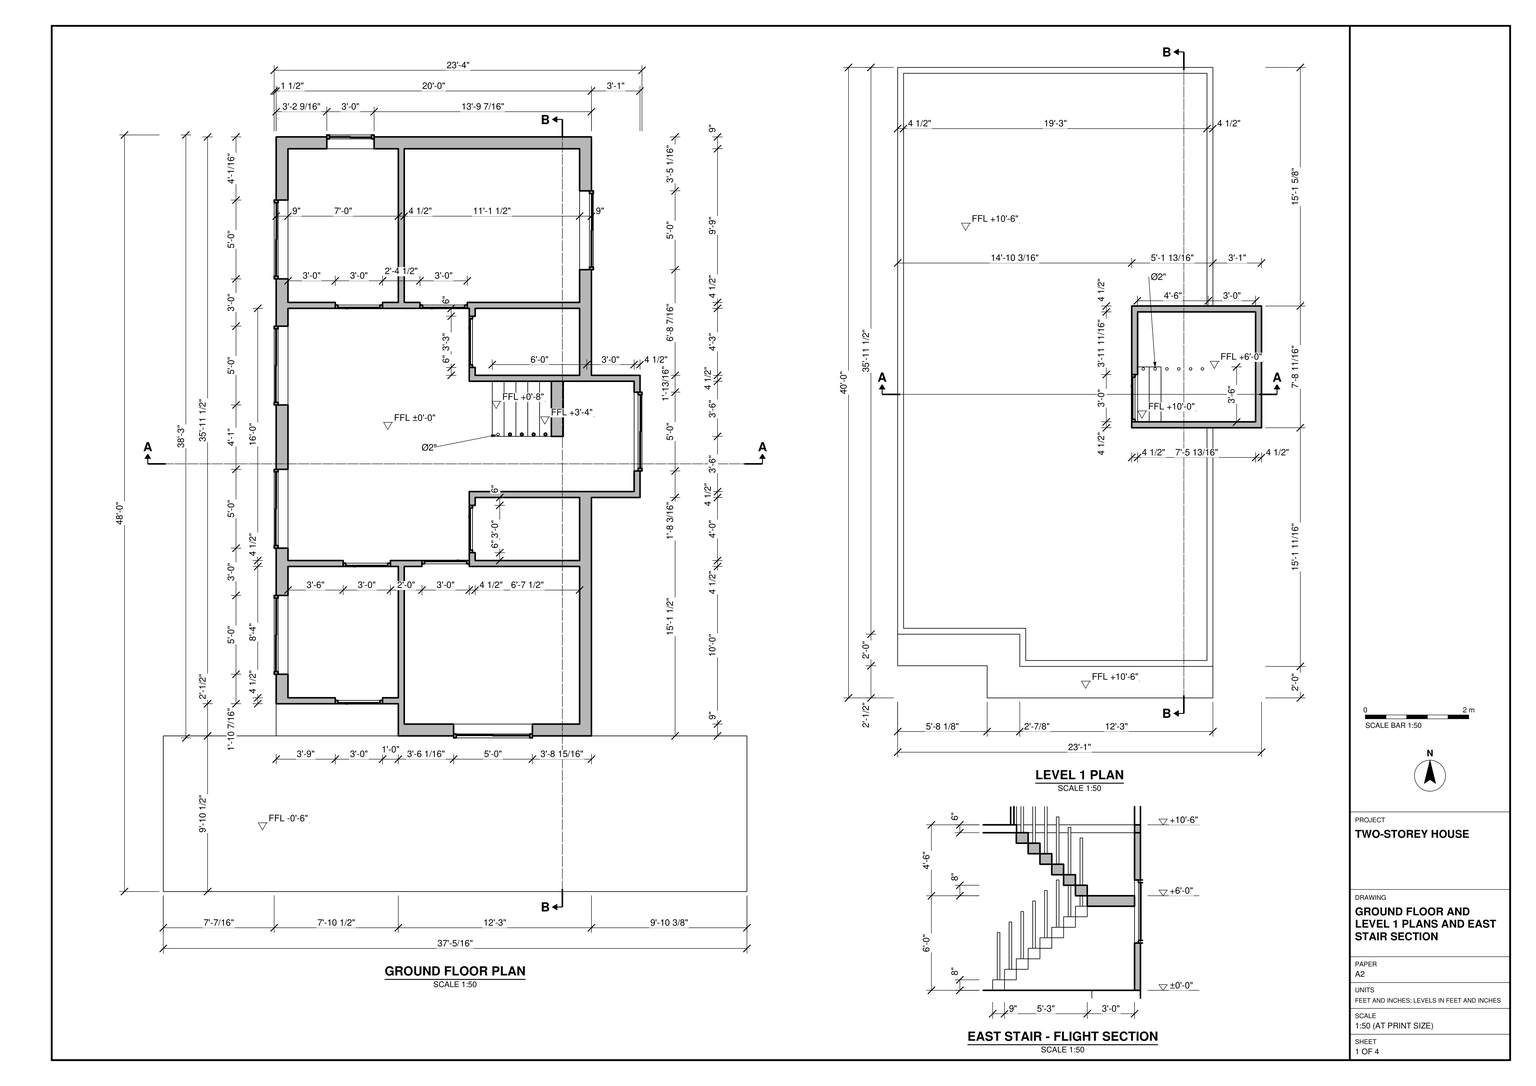
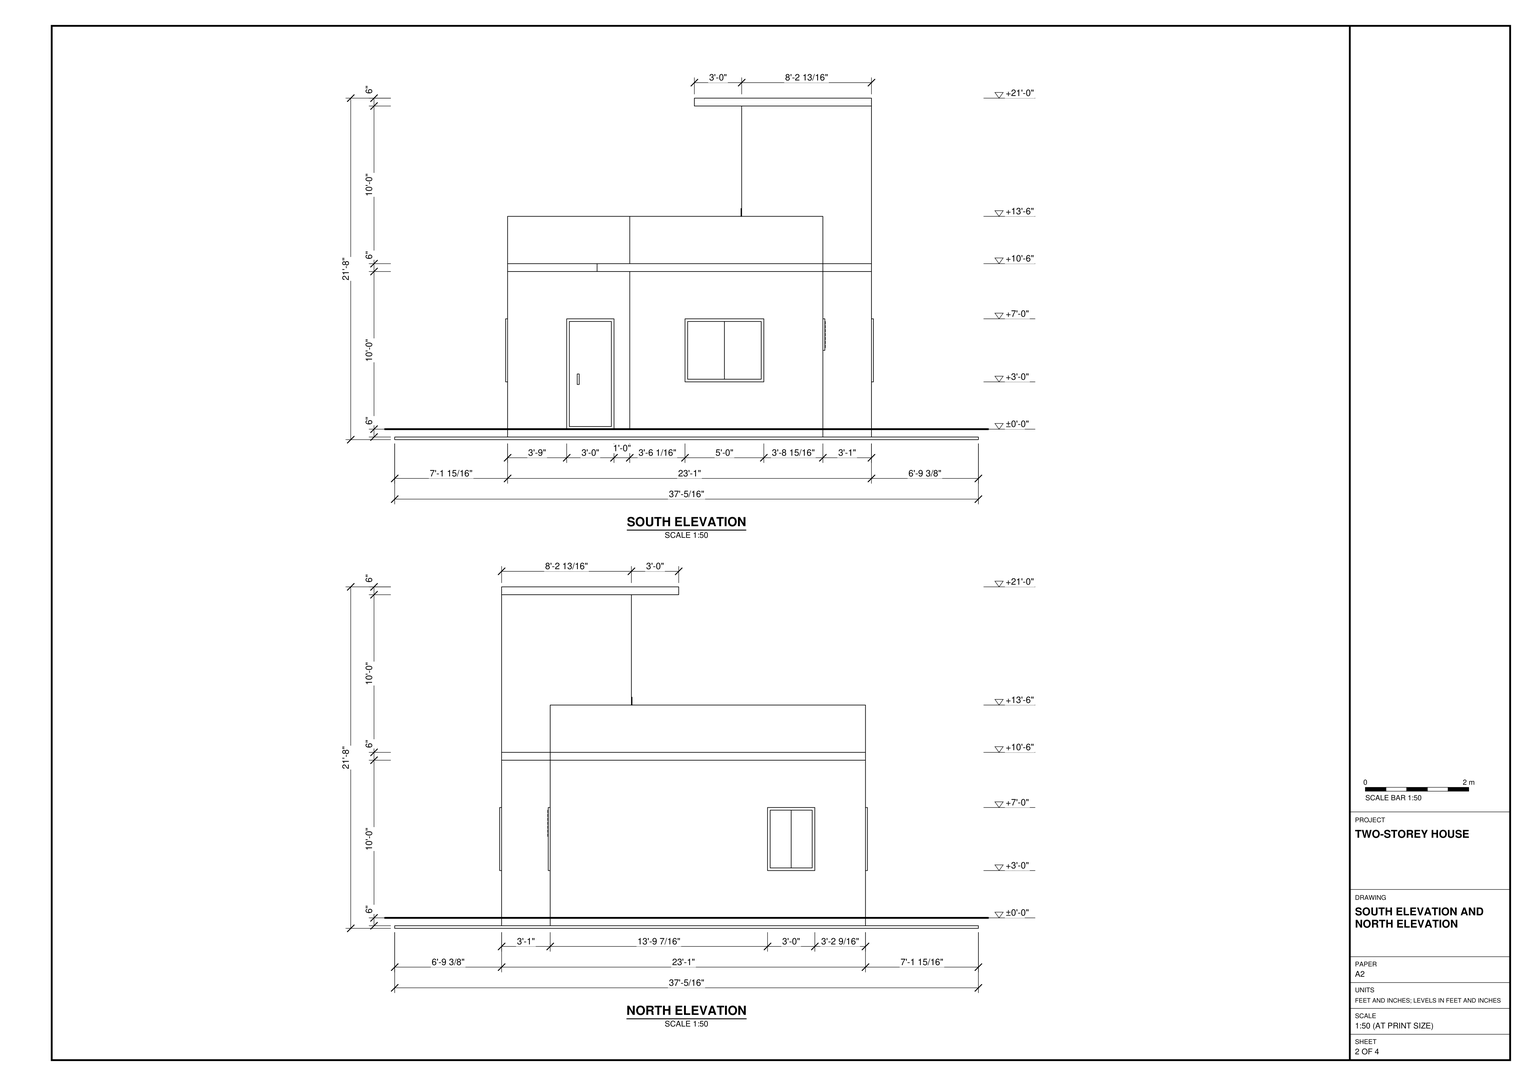
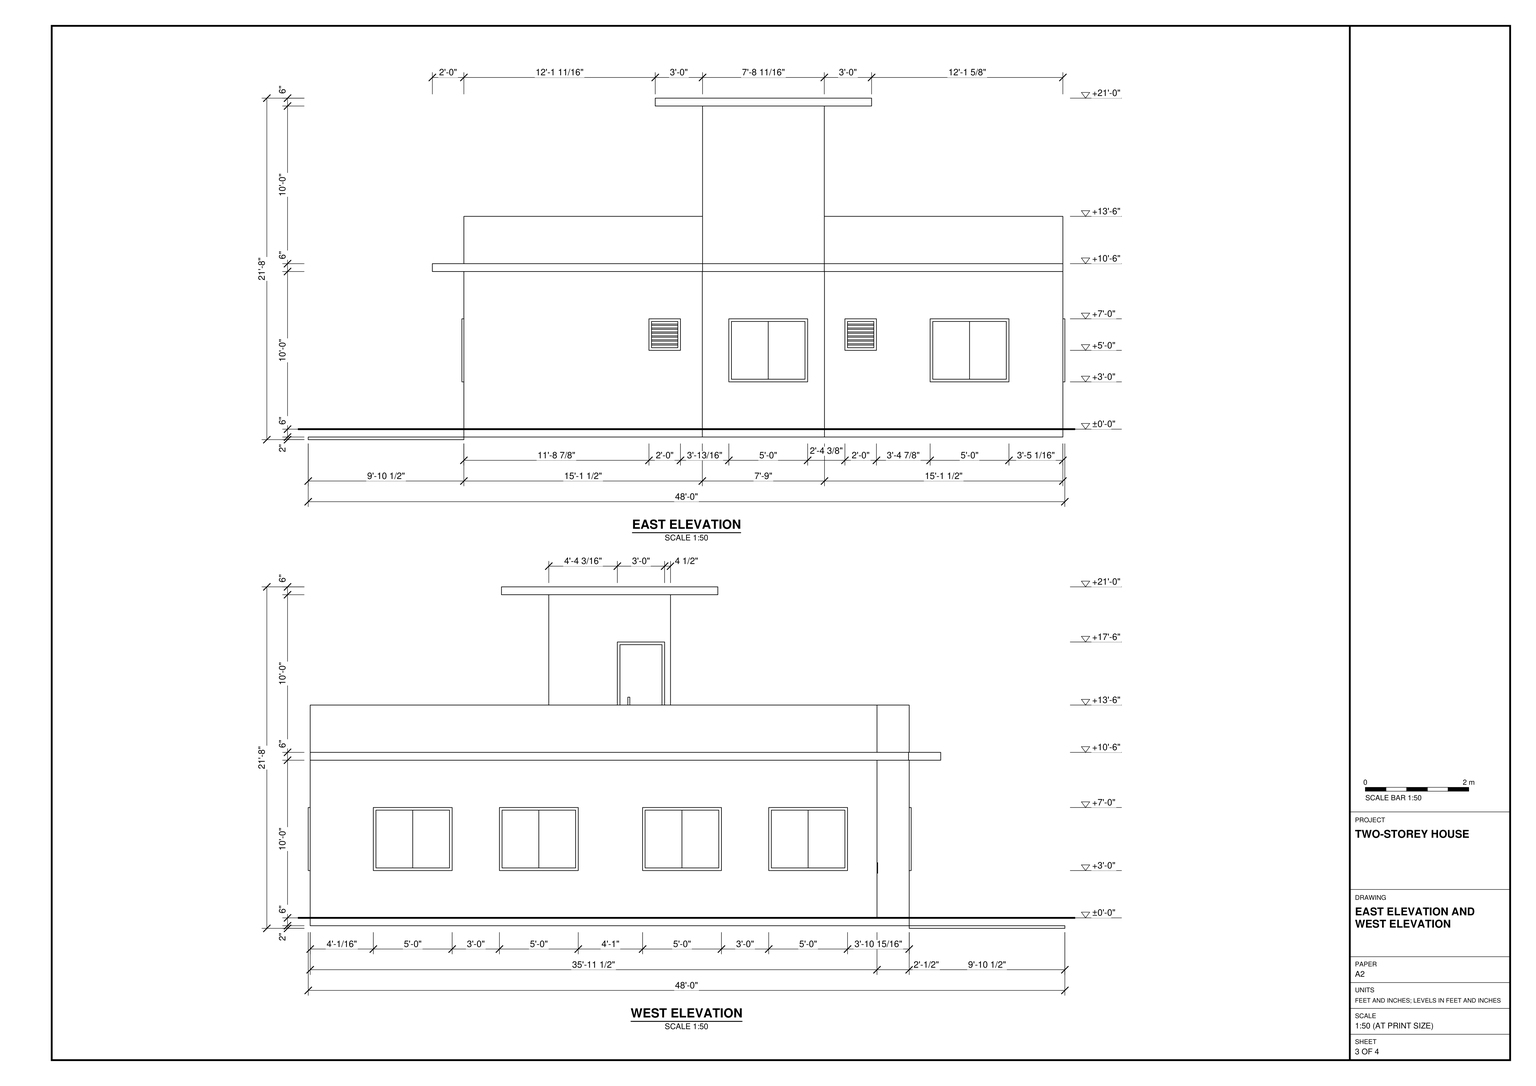
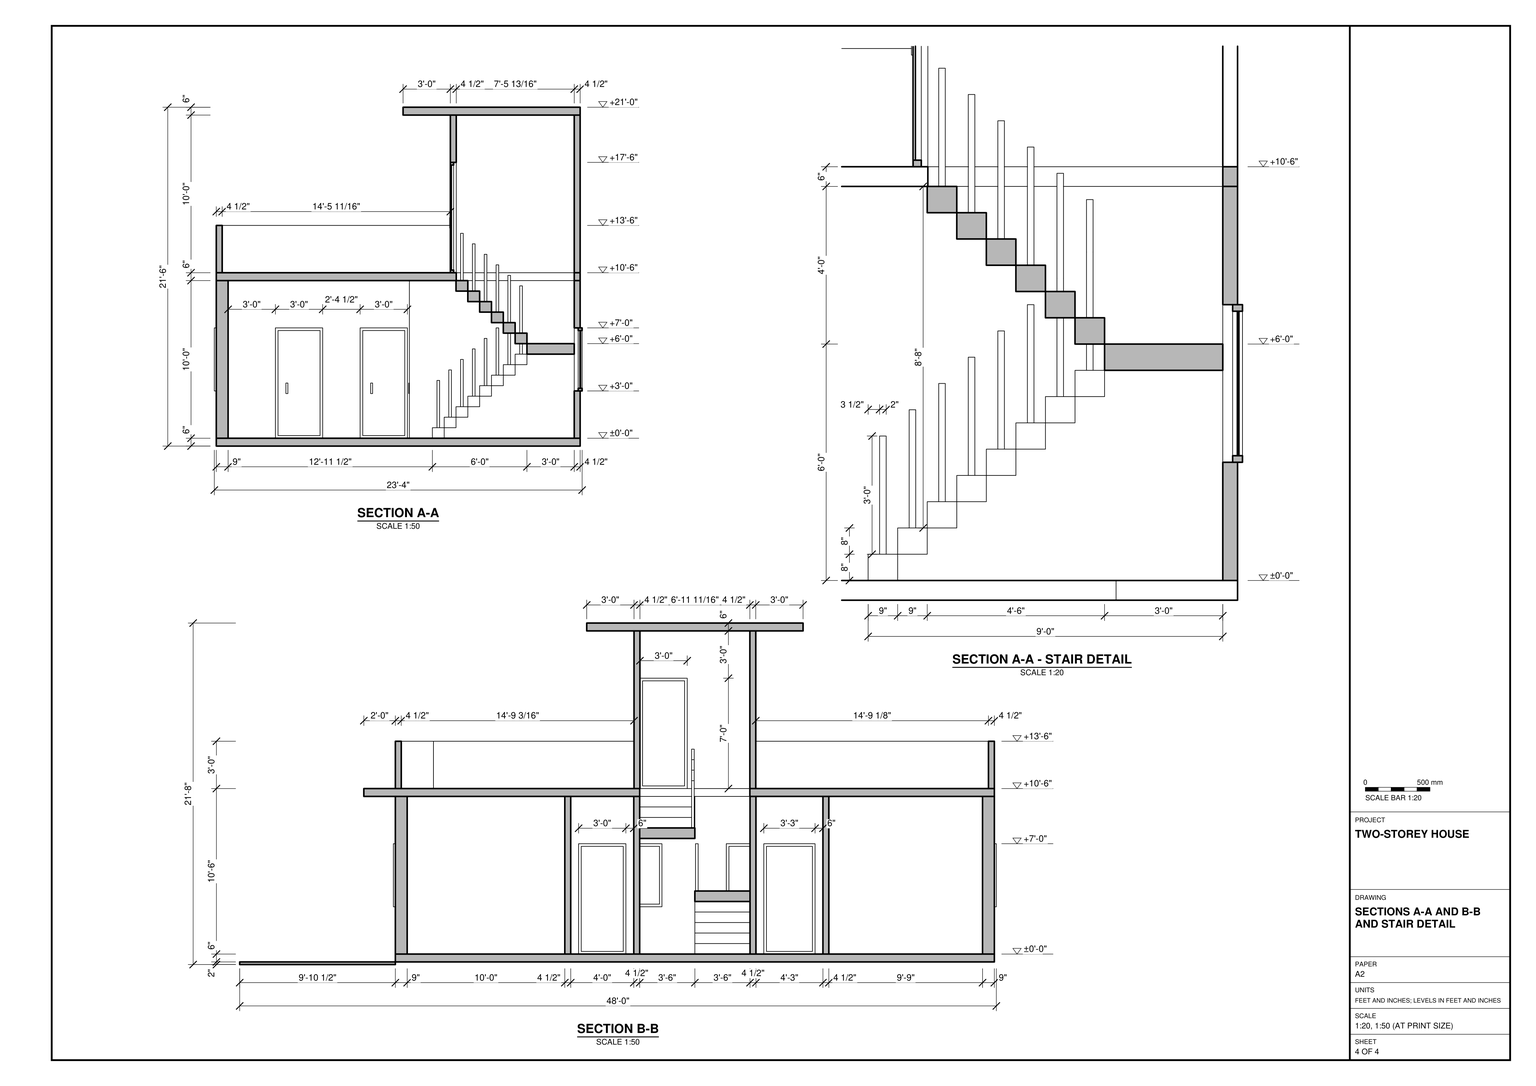
Build the house in SketchUp from task_files/diagram_01.pdf, working in feet and inches. Including the base, the overall model is 37'-5/16" east to west, 48'-0" north to south and 21'-8" high. Set the ground-floor finished level at ±0'-0" and the upper terrace at +10'-6".

Use the ground-floor plan to position the house behind the front forecourt. Follow the stepped south frontage and the projecting stair bay on the east. Model the main exterior walls at 9" thick and the partitions at 4 1/2" thick where indicated. Lay out the paired rooms at the north and south ends, the central space and the small rooms on either side of the stair. Use the plans to locate doorways and the elevations to set window widths, sills and heads. Distinguish the small louvred east openings from the larger glazed windows.

Build the stair flights and intermediate landing from the stair section. Form the upper slab around the stair opening, with a parapet around the terrace and a west-facing door from the stair enclosure. Give the enclosure its own overhanging flat roof. Keep walls, slabs, stairs and roof elements in separate groups or components. Keep each furniture or joinery piece separate if shown, and use components for repeated parts. Any decor or loose items may be suitable library components. Save one SketchUp model as output_files/two_storey_house_with_an_east_stair_and_roof_terrace.skp.

# SketchUp Ruby script. Lengths in inches.
U = 1.inch
M = Sketchup.active_model
def pt(a) = Geom::Point3d.new(a.map { |v| v * U })
def face(e, loops, mat)
  f = e.add_face(loops[0].map { |a| pt(a) })
  loops[1..].each { |l| e.add_face(l.map { |a| pt(a) }).erase! }
  f.material = f.back_material = mat if mat
  f
end
# faces: each face lists its corners as indices into pts; further lists are holes
def faces(e, pts, list, mat = nil) = list.each { |f| face(e, (f[0].is_a?(Array) ? f : [f]).map { |l| l.map { |i| pts[i] } }, mat) }
# xy, xz, yz: faces in a plane at the given z, y or x. An outline is a flat list of corners, or four numbers for a rectangle; further outlines are holes
def ring(l) = l.size == 4 ? [[l[0], l[1]], [l[2], l[1]], [l[2], l[3]], [l[0], l[3]]] : l.each_slice(2).to_a
def flat(e, list, mat, &to3) = list.each { |f| face(e, (f[0].is_a?(Array) ? f : [f]).map { |l| ring(l).map { |u, v| to3.(u, v) } }, mat) }
def xy(e, z, list, mat = nil) = flat(e, list, mat) { |x, y| [x, y, z] }
def xz(e, y, list, mat = nil) = flat(e, list, mat) { |x, z| [x, y, z] }
def yz(e, x, list, mat = nil) = flat(e, list, mat) { |y, z| [x, y, z] }
def lines(e, pts, list) = list.each { |a, b| e.add_line(pt(pts[a]), pt(pts[b])) }
# prism: a flat outline (further loops are holes) pulled along v
def prism(e, loops, v, mat = nil)
  f = face(e, loops, mat); d = Geom::Vector3d.new(v.map { |x| x * U })
  f.pushpull(f.normal.samedirection?(d) ? d.length : -d.length)
end
def box(e, o, s, mat = nil) = prism(e, [[o, [o[0] + s[0], o[1], o[2]], [o[0] + s[0], o[1] + s[1], o[2]], [o[0], o[1] + s[1], o[2]]]], [0, 0, s[2]], mat)
def at(x, y, z, deg = 0) = Geom::Transformation.translation(pt([x, y, z])) * Geom::Transformation.rotation(ORIGIN, Z_AXIS, deg.degrees)
def axes(o, x, y, z) = Geom::Transformation.new([*x, 0, *y, 0, *z, 0, *pt(o).to_a, 1])
def part(name) = M.definitions.add(name)
# library, detail: a bought-in or finely detailed component or shape, given as its bounding box
def library(name, o, s) = part(name).tap { |d| box(d.entities, o, s) }
def detail(e, o, s) = box(e.add_group.entities, o, s)
def put(e, d, t, mat = nil) = e.add_instance(d, t).tap { |i| i.material = mat if mat }
def group(e, t, mat = nil) = e.add_group.tap { |g| g.transformation = t; g.material = mat if mat }.entities
root = M.entities
M.materials.add("Asphalt A02 100cm").color = [81, 81, 83]
M.materials.add("Glass Yellow 001").color = [0, 0, 0]
M.materials["Glass Yellow 001"].alpha = 0.1
M.materials.add("Marble Black 100cm").color = [32, 32, 32]
M.materials.add("Metal Sandblasted Black 200cm").color = [86, 90, 95]
M.materials.add("Two Color Maple Panels 300cm").color = [56, 46, 41]
M.materials.add("Wall Paint Fine Grain 01 Yellow 100cm").color = [207, 190, 139]
M.materials.add("Wall Paint Poised Taupe Satin 300cm").color = [140, 135, 132]
c1 = part("Group\#3")
box(c1.entities,[0,0,0],[0.31,28,44])
c2 = part("Group\#5")
box(c2.entities,[0,0,0],[0.31,28,44])
c3 = part("Group\#7")
box(c3.entities,[0,0,0],[0.31,28.0625,44])
c4 = part("Group\#9")
box(c4.entities,[0,0,0],[0.31,28,44])
c5 = part("Group\#11")
box(c5.entities,[0,0,0],[28,0.31,44])
c6 = part("Group\#13")
box(c6.entities,[0,0,0],[0.31,20,2])
c7 = part("Group\#15")
box(c7.entities,[-0.31,0,0],[0.31,28,44])
c8 = part("Group\#17")
box(c8.entities,[0,0,0],[0.31,20,2])
c9 = part("Group\#19")
box(c9.entities,[-0.31,0,0],[0.31,28,44])
c10 = part("Group\#21")
box(c10.entities,[0,-0.31,0],[16,0.31,44])
xy(root,135.74,[[154.0625,94.5,325.9375,94.5,325.9375,118.5,178.9375,118.5,178.9375,143,85.9375,143,85.9375,119,154.0625,119]])
g1 = group(root,at(85.9375,118.5,9.74))
xy(g1,0,[[0,0,93,0,93,24.5,81,24.5,81,29,93,29,93,129,87,129,87,133.5,111,133.5,111,129,97.5,129,97.5,9,231,9,231,129,147,129,147,139.5,151.5,139.5,151.5,133.5,231,133.5,231,181.5,151.5,181.5,151.5,175.5,147,175.5,147,186,272.5,186,272.5,270,147,270,147,280.5,151.5,280.5,151.5,274.5,231,274.5,231,325.5,151.5,325.5,151.5,319.5,147,319.5,147,325.5,145.5,325.5,145.5,330,231,330,231,447,97.5,447,97.5,330,109.5,330,109.5,325.5,81,325.5,81,330,93,330,93,447,9,447,9,330,45,330,45,325.5,9,325.5,9,133.5,51,133.5,51,129,9,129,9,29,45,29,45,24.5,0,24.5]],"Wall Paint Fine Grain 01 Yellow 100cm")
xy(g1,36,[[135.0625,0,195.0625,9],[0,46.9375,9,106.9375],[0,142.9375,9,202.9375],[272.5,201.6875,277,261.6875],[0,251.9375,9,311.9375],
  [0,347.9375,9,407.9375],[231,354.9375,240,414.9375],[38.5625,447,74.5625,456]],"Wall Paint Fine Grain 01 Yellow 100cm")
xy(g1,60,[[231,140.875,240,164.875],[231,290.0625,240,314.0625]],"Wall Paint Fine Grain 01 Yellow 100cm")
xy(g1,84,[[135.0625,0,195.0625,9],[45,24.5,81,29],[0,46.9375,9,106.9375],[51,129,87,133.5],[111,129,147,133.5],
  [147,139.5,151.5,175.5],[231,140.875,240,164.875],[0,142.9375,9,202.9375],[272.5,201.6875,277,261.6875],[0,251.9375,9,311.9375],
  [147,280.5,151.5,319.5],[231,290.0625,240,314.0625],[45,325.5,81,330],[109.5,325.5,145.5,330],[0,347.9375,9,407.9375],
  [231,354.9375,240,414.9375],[38.5625,447,74.5625,456]],"Wall Paint Fine Grain 01 Yellow 100cm")
xy(g1,120,[[[93,0,240,0,240,181.5,277,181.5,277,274.5,240,274.5,240,456,0,456,0,24.5,93,24.5],[9,133.5,9,325.5,147,325.5,147,270,272.5,270,272.5,186,147,186,147,133.5],[97.5,9,231,129],[97.5,330,231,447],[9,330,93,447],[9,29,93,129],[151.5,274.5,231,325.5],[151.5,133.5,231,181.5]]],"Wall Paint Fine Grain 01 Yellow 100cm")
xz(g1,0,[[[93,0,240,120],[135.0625,36,195.0625,84]]],"Wall Paint Fine Grain 01 Yellow 100cm")
xz(g1,9,[[[97.5,0,231,120],[135.0625,36,195.0625,84]]],"Wall Paint Fine Grain 01 Yellow 100cm")
xz(g1,24.5,[[0,0,45,0,45,84,81,84,81,0,93,0,93,120,0,120]],"Wall Paint Fine Grain 01 Yellow 100cm")
xz(g1,29,[[9,0,9,120,93,120,93,0,81,0,81,84,45,84,45,0]],"Wall Paint Fine Grain 01 Yellow 100cm")
xz(g1,46.9375,[[0,36,9,84]],"Wall Paint Fine Grain 01 Yellow 100cm")
xz(g1,106.9375,[[0,36,9,84]],"Wall Paint Fine Grain 01 Yellow 100cm")
xz(g1,129,[[9,0,51,0,51,84,87,84,87,0,93,0,93,120,9,120],[97.5,0,111,0,111,84,147,84,147,0,231,0,231,120,97.5,120]],"Wall Paint Fine Grain 01 Yellow 100cm")
xz(g1,133.5,[[9,0,9,120,147,120,147,84,111,84,111,0,87,0,87,84,51,84,51,0],[151.5,0,231,120]],"Wall Paint Fine Grain 01 Yellow 100cm")
xz(g1,139.5,[[147,0,151.5,84]],"Wall Paint Fine Grain 01 Yellow 100cm")
xz(g1,140.875,[[231,60,240,84]],"Wall Paint Fine Grain 01 Yellow 100cm")
xz(g1,142.9375,[[0,36,9,84]],"Wall Paint Fine Grain 01 Yellow 100cm")
xz(g1,164.875,[[231,60,240,84]],"Wall Paint Fine Grain 01 Yellow 100cm")
xz(g1,175.5,[[147,0,151.5,84]],"Wall Paint Fine Grain 01 Yellow 100cm")
xz(g1,181.5,[[151.5,0,231,120],[240,0,277,120]],"Wall Paint Fine Grain 01 Yellow 100cm")
xz(g1,186,[[147,0,272.5,120]],"Wall Paint Fine Grain 01 Yellow 100cm")
xz(g1,201.6875,[[272.5,36,277,84]],"Wall Paint Fine Grain 01 Yellow 100cm")
xz(g1,202.9375,[[0,36,9,84]],"Wall Paint Fine Grain 01 Yellow 100cm")
xz(g1,251.9375,[[0,36,9,84]],"Wall Paint Fine Grain 01 Yellow 100cm")
xz(g1,261.6875,[[272.5,36,277,84]],"Wall Paint Fine Grain 01 Yellow 100cm")
xz(g1,270,[[147,0,272.5,120]],"Wall Paint Fine Grain 01 Yellow 100cm")
xz(g1,274.5,[[151.5,0,231,120],[240,0,277,120]],"Wall Paint Fine Grain 01 Yellow 100cm")
xz(g1,280.5,[[147,0,151.5,84]],"Wall Paint Fine Grain 01 Yellow 100cm")
xz(g1,290.0625,[[231,60,240,84]],"Wall Paint Fine Grain 01 Yellow 100cm")
xz(g1,311.9375,[[0,36,9,84]],"Wall Paint Fine Grain 01 Yellow 100cm")
xz(g1,314.0625,[[231,60,240,84]],"Wall Paint Fine Grain 01 Yellow 100cm")
xz(g1,319.5,[[147,0,151.5,84]],"Wall Paint Fine Grain 01 Yellow 100cm")
xz(g1,325.5,[[9,0,45,0,45,84,81,84,81,0,109.5,0,109.5,84,145.5,84,145.5,0,147,0,147,120,9,120],[151.5,0,231,120]],"Wall Paint Fine Grain 01 Yellow 100cm")
xz(g1,330,[[9,0,9,120,93,120,93,0,81,0,81,84,45,84,45,0],[97.5,0,97.5,120,231,120,231,0,145.5,0,145.5,84,109.5,84,109.5,0]],"Wall Paint Fine Grain 01 Yellow 100cm")
xz(g1,347.9375,[[0,36,9,84]],"Wall Paint Fine Grain 01 Yellow 100cm")
xz(g1,354.9375,[[231,36,240,84]],"Wall Paint Fine Grain 01 Yellow 100cm")
xz(g1,407.9375,[[0,36,9,84]],"Wall Paint Fine Grain 01 Yellow 100cm")
xz(g1,414.9375,[[231,36,240,84]],"Wall Paint Fine Grain 01 Yellow 100cm")
xz(g1,447,[[[9,0,93,120],[38.5625,36,74.5625,84]],[97.5,0,231,120]],"Wall Paint Fine Grain 01 Yellow 100cm")
xz(g1,456,[[[0,0,240,120],[38.5625,36,74.5625,84]]],"Wall Paint Fine Grain 01 Yellow 100cm")
yz(g1,0,[[[24.5,0,456,120],[46.9375,36,106.9375,84],[251.9375,36,311.9375,84],[142.9375,36,202.9375,84],[347.9375,36,407.9375,84]]],"Wall Paint Fine Grain 01 Yellow 100cm")
yz(g1,9,[[[29,0,129,120],[46.9375,36,106.9375,84]],[[133.5,0,325.5,120],[251.9375,36,311.9375,84],[142.9375,36,202.9375,84]],[[330,0,447,120],[347.9375,36,407.9375,84]]],"Wall Paint Fine Grain 01 Yellow 100cm")
yz(g1,38.5625,[[447,36,456,84]],"Wall Paint Fine Grain 01 Yellow 100cm")
yz(g1,45,[[24.5,0,29,84],[325.5,0,330,84]],"Wall Paint Fine Grain 01 Yellow 100cm")
yz(g1,51,[[129,0,133.5,84]],"Wall Paint Fine Grain 01 Yellow 100cm")
yz(g1,74.5625,[[447,36,456,84]],"Wall Paint Fine Grain 01 Yellow 100cm")
yz(g1,81,[[24.5,0,29,84],[325.5,0,330,84]],"Wall Paint Fine Grain 01 Yellow 100cm")
yz(g1,87,[[129,0,133.5,84]],"Wall Paint Fine Grain 01 Yellow 100cm")
yz(g1,93,[[0,0,24.5,120],[29,0,129,120],[330,0,447,120]],"Wall Paint Fine Grain 01 Yellow 100cm")
yz(g1,97.5,[[9,0,129,120],[330,0,447,120]],"Wall Paint Fine Grain 01 Yellow 100cm")
yz(g1,109.5,[[325.5,0,330,84]],"Wall Paint Fine Grain 01 Yellow 100cm")
yz(g1,111,[[129,0,133.5,84]],"Wall Paint Fine Grain 01 Yellow 100cm")
yz(g1,135.0625,[[0,36,9,84]],"Wall Paint Fine Grain 01 Yellow 100cm")
yz(g1,145.5,[[325.5,0,330,84]],"Wall Paint Fine Grain 01 Yellow 100cm")
yz(g1,147,[[129,0,129,84,133.5,84,133.5,120,186,120,186,0,175.5,0,175.5,84,139.5,84,139.5,0],[270,0,270,120,325.5,120,325.5,0,319.5,0,319.5,84,280.5,84,280.5,0]],"Wall Paint Fine Grain 01 Yellow 100cm")
yz(g1,151.5,[[133.5,0,139.5,0,139.5,84,175.5,84,175.5,0,181.5,0,181.5,120,133.5,120],[274.5,0,280.5,0,280.5,84,319.5,84,319.5,0,325.5,0,325.5,120,274.5,120]],"Wall Paint Fine Grain 01 Yellow 100cm")
yz(g1,195.0625,[[0,36,9,84]],"Wall Paint Fine Grain 01 Yellow 100cm")
yz(g1,231,[[9,0,129,120],[[133.5,0,181.5,120],[140.875,60,164.875,84]],[[274.5,0,325.5,120],[290.0625,60,314.0625,84]],[[330,0,447,120],[354.9375,36,414.9375,84]]],"Wall Paint Fine Grain 01 Yellow 100cm")
yz(g1,240,[[[0,0,181.5,120],[140.875,60,164.875,84]],[[274.5,0,456,120],[354.9375,36,414.9375,84],[290.0625,60,314.0625,84]]],"Wall Paint Fine Grain 01 Yellow 100cm")
yz(g1,272.5,[[[186,0,270,120],[201.6875,36,261.6875,84]]],"Wall Paint Fine Grain 01 Yellow 100cm")
yz(g1,277,[[[181.5,0,274.5,120],[201.6875,36,261.6875,84]]],"Wall Paint Fine Grain 01 Yellow 100cm")
g2 = group(g1,at(0,347.9375,36))
prism(g2,[[[-1.5,60,0],[-1.5,0,0],[-1.5,0,48],[-1.5,60,48]],[[-1.5,2,46],[-1.5,2,2],[-1.5,58,2],[-1.5,58,46]]],[3,0,0],"Metal Sandblasted Black 200cm")
put(g2,c1,at(0.125,30,2),"Glass Yellow 001")
put(g2,c1,at(-0.19,2,2),"Glass Yellow 001")
g3 = group(g1,at(0,251.9375,36))
prism(g3,[[[-1.5,60,0],[-1.5,0,0],[-1.5,0,48],[-1.5,60,48]],[[-1.5,2,2],[-1.5,58,2],[-1.5,58,46],[-1.5,2,46]]],[3,0,0],"Metal Sandblasted Black 200cm")
put(g3,c2,at(-0.1875,30,2),"Glass Yellow 001")
put(g3,c2,at(-0.5,2,2),"Glass Yellow 001")
g4 = group(g1,at(0,142.9375,36))
prism(g4,[[[-1.5,60,0],[-1.5,0,0],[-1.5,0,48],[-1.5,60,48]],[[-1.5,2,46],[-1.5,2,2],[-1.5,58.125,2],[-1.5,58.125,46]]],[3,0,0],"Metal Sandblasted Black 200cm")
put(g4,c3,at(-0.25,30.0625,2),"Glass Yellow 001")
put(g4,c3,at(-0.56,2,2),"Glass Yellow 001")
g5 = group(g1,at(0,46.9375,36))
prism(g5,[[[-1.5,0,0],[-1.5,0,48],[-1.5,60,48],[-1.5,60,0]],[[-1.5,2,46],[-1.5,2,2],[-1.5,58,2],[-1.5,58,46]]],[3,0,0],"Metal Sandblasted Black 200cm")
put(g5,c4,at(-0.0625,30,2),"Glass Yellow 001")
put(g5,c4,at(-0.38,2,2),"Glass Yellow 001")
g6 = group(g1,at(135.0625,0,36))
prism(g6,[[[60,-1.5,0],[60,-1.5,48],[0,-1.5,48],[0,-1.5,0]],[[58,-1.5,46],[58,-1.5,2],[2,-1.5,2],[2,-1.5,46]]],[0,3,0],"Metal Sandblasted Black 200cm")
put(g6,c5,at(2,0.4375,2),"Glass Yellow 001")
put(g6,c5,at(30,0.12,2),"Glass Yellow 001")
g7 = group(g1,at(240,140.875,60))
prism(g7,[[[1.5,0,0],[1.5,24,0],[1.5,24,24],[1.5,0,24]],[[1.5,22,2],[1.5,2,2],[1.5,2,22],[1.5,22,22]]],[-3,0,0],"Metal Sandblasted Black 200cm")
put(g7,c6,at(1.5,2,20),"Glass Yellow 001")
put(g7,c6,at(1.5,2,17),"Glass Yellow 001")
put(g7,c6,at(1.5,2,14),"Glass Yellow 001")
put(g7,c6,at(1.5,2,11),"Glass Yellow 001")
put(g7,c6,at(1.5,2,8),"Glass Yellow 001")
put(g7,c6,at(1.5,2,5),"Glass Yellow 001")
put(g7,c6,at(1.5,2,2),"Glass Yellow 001")
g8 = group(g1,at(277,201.6875,36))
prism(g8,[[[1.5,0,0],[1.5,60,0],[1.5,60,48],[1.5,0,48]],[[1.5,58,2],[1.5,2,2],[1.5,2,46],[1.5,58,46]]],[-3,0,0],"Metal Sandblasted Black 200cm")
put(g8,c7,at(0.25,2,2),"Glass Yellow 001")
put(g8,c7,at(0.56,30,2),"Glass Yellow 001")
g9 = group(g1,at(240,290.0625,60))
prism(g9,[[[1.5,0,0],[1.5,24,0],[1.5,24,24],[1.5,0,24]],[[1.5,22,2],[1.5,2,2],[1.5,2,22],[1.5,22,22]]],[-3,0,0],"Metal Sandblasted Black 200cm")
put(g9,c8,at(1.5,2,20),"Glass Yellow 001")
put(g9,c8,at(1.5,2,17),"Glass Yellow 001")
put(g9,c8,at(1.5,2,14),"Glass Yellow 001")
put(g9,c8,at(1.5,2,11),"Glass Yellow 001")
put(g9,c8,at(1.5,2,8),"Glass Yellow 001")
put(g9,c8,at(1.5,2,5),"Glass Yellow 001")
put(g9,c8,at(1.5,2,2),"Glass Yellow 001")
g10 = group(g1,at(240,354.9375,36))
prism(g10,[[[1.5,0,0],[1.5,60,0],[1.5,60,48],[1.5,0,48]],[[1.5,58,46],[1.5,58,2],[1.5,2,2],[1.5,2,46]]],[-3,0,0],"Metal Sandblasted Black 200cm")
put(g10,c9,at(0.25,2,2),"Glass Yellow 001")
put(g10,c9,at(0.56,30,2),"Glass Yellow 001")
g11 = group(g1,at(38.5625,456,36))
prism(g11,[[[0,1.5,0],[0,1.5,48],[36,1.5,48],[36,1.5,0]],[[34,1.5,2],[34,1.5,46],[2,1.5,46],[2,1.5,2]]],[0,-3,0],"Metal Sandblasted Black 200cm")
put(g11,c10,at(18,-0.1875,2),"Glass Yellow 001")
put(g11,c10,at(2,0.13,2),"Glass Yellow 001")
g12 = group(g1,at(45,24.5,0))
prism(g12,[[[36,0,0],[36,0,84],[0,0,84],[0,0,0]],[[2,0,82],[34,0,82],[34,0,2],[2,0,2]]],[0,2.5,0],"Metal Sandblasted Black 200cm")
g13 = group(g12,at(2,0,2))
box(g13,[0,0,0],[32,0.71,80],"Two Color Maple Panels 300cm")
g14 = group(g12,at(8,0,34))
box(g14,[0,-0.5,0],[1.5,0.5,8],"Metal Sandblasted Black 200cm")
g15 = group(g1,at(51,129,0))
prism(g15,[[[36,0,0],[36,0,84],[0,0,84],[0,0,0]],[[2,0,2],[2,0,82],[34,0,82],[34,0,2]]],[0,2.5,0])
g16 = group(g15,at(2,0,2))
box(g16,[0,0,0],[32,0.71,80])
g17 = group(g16,at(6,0,32))
box(g17,[0,-0.5,0],[1.5,0.5,8])
g18 = group(g1,at(111,133.5,0))
prism(g18,[[[0,0,0],[0,0,84],[36,0,84],[36,0,0]],[[34,0,2],[34,0,82],[2,0,82],[2,0,2]]],[0,-2.5,0])
g19 = group(g18,at(2,0,2))
box(g19,[0,-0.71,0],[32,0.71,80])
g20 = group(g19,at(26,0,32))
box(g20,[-1.5,0,0],[1.5,0.5,8])
g21 = group(g1,at(147,139.5,0))
prism(g21,[[[0,0,0],[0,0,84],[0,36,84],[0,36,0]],[[0,34,2],[0,34,82],[0,2,82],[0,2,2]]],[2.5,0,0])
g22 = group(g21,at(0,2,2))
box(g22,[0,0,0],[0.71,32,80])
g23 = group(g22,at(0,26,32))
box(g23,[-0.5,-1.5,0],[0.5,1.5,8])
g24 = group(g1,at(147,280.5,0))
prism(g24,[[[0,0,0],[0,0,84],[0,39,84],[0,39,0]],[[0,2,82],[0,2,2],[0,37,2],[0,37,82]]],[2.5,0,0])
g25 = group(g24,at(0,2,2))
box(g25,[0,0,0],[0.71,35,80])
g26 = group(g25,at(0,29,32))
box(g26,[-0.5,-1.5,0],[0.5,1.5,8])
g27 = group(g1,at(45,325.5,0))
prism(g27,[[[36,0,0],[36,0,84],[0,0,84],[0,0,0]],[[2,0,2],[2,0,82],[34,0,82],[34,0,2]]],[0,2.5,0])
g28 = group(g27,at(2,0,2))
box(g28,[0,0,0],[32,0.71,80])
g29 = group(g28,at(6,0,32))
box(g29,[0,-0.5,0],[1.5,0.5,8])
g30 = group(g1,at(109.5,325.5,0))
prism(g30,[[[36,0,0],[36,0,84],[0,0,84],[0,0,0]],[[34,0,82],[34,0,2],[2,0,2],[2,0,82]]],[0,2.5,0])
g31 = group(g30,at(2,0,2))
box(g31,[0,0,0],[32,0.71,80])
g32 = group(g31,at(6,0,32))
box(g32,[0,-0.5,0],[1.5,0.5,8])
g33 = group(root,at(85.9375,143,129.74))
xy(g33,0,[[[68.125,-48.5,68.125,-24,0,-24,0,431.5,240,431.5,240,249.875,277,249.875,277,157.1875,240,157.1875,240,-48.5],[182.69,161.5,272.5,245.375]]],"Marble Black 100cm")
xy(g33,6,[[97.5,-20,235.5,-20,235.5,161.5,182.69,161.5,182.69,245.375,235.5,245.375,235.5,427,4.5,427,4.5,4.5,97.5,4.5]],"Marble Black 100cm")
xz(g33,-48.5,[[68.125,0,240,6]],"Marble Black 100cm")
xz(g33,-24,[[0,0,68.125,6]],"Marble Black 100cm")
xz(g33,157.1875,[[240,0,277,6]],"Marble Black 100cm")
xz(g33,161.5,[[182.69,0,272.5,6]],"Marble Black 100cm")
xz(g33,245.375,[[182.69,0,272.5,6]],"Marble Black 100cm")
xz(g33,249.875,[[240,0,277,6]],"Marble Black 100cm")
xz(g33,431.5,[[0,0,240,6]],"Marble Black 100cm")
yz(g33,0,[[-24,0,431.5,6]],"Marble Black 100cm")
yz(g33,68.125,[[-48.5,0,-24,6]],"Marble Black 100cm")
yz(g33,182.69,[[161.5,0,245.375,6]],"Marble Black 100cm")
yz(g33,240,[[-48.5,0,157.1875,6],[249.875,0,431.5,6]],"Marble Black 100cm")
yz(g33,272.5,[[161.5,0,245.375,6]],"Marble Black 100cm")
yz(g33,277,[[157.1875,0,249.875,6]],"Marble Black 100cm")
g34 = group(g33,at(0,-24.5,6))
xy(g34,0,[[[93,0,93,24.5,0,24.5,0,456,240,456,240,274.375,277,274.375,277,181.6875,240,181.6875,240,0],[97.5,4.5,235.5,4.5,235.5,181.6875,178.19,181.6875,178.19,186.1875,272.5,186.1875,272.5,269.875,182.69,269.875,182.69,222.1875,178.19,222.1875,178.19,274.375,235.5,274.375,235.5,451.5,4.5,451.5,4.5,29,97.5,29]]])
xy(g34,36,[[93,0,240,0,240,181.6875,235.5,181.6875,235.5,4.5,97.5,4.5,97.5,29,4.5,29,4.5,451.5,235.5,451.5,235.5,274.375,240,274.375,240,456,0,456,0,24.5,93,24.5]])
xy(g34,84,[[178.19,186.1875,182.69,222.1875]])
xy(g34,120,[[[178.19,181.6875,277,274.375],[182.69,186.1875,272.5,269.875]]])
xz(g34,0,[[93,0,240,36]],"Wall Paint Poised Taupe Satin 300cm")
xz(g34,4.5,[[97.5,0,235.5,36]])
xz(g34,24.5,[[0,0,93,36]],"Wall Paint Poised Taupe Satin 300cm")
xz(g34,29,[[4.5,0,97.5,36]])
xz(g34,181.6875,[[178.19,0,235.5,0,235.5,36,240,36,240,0,277,0,277,120,178.19,120]],"Wall Paint Fine Grain 01 Yellow 100cm")
xz(g34,186.1875,[[178.19,0,178.19,84,182.69,84,182.69,120,272.5,120,272.5,0]])
xz(g34,222.1875,[[178.19,0,182.69,84]])
xz(g34,269.875,[[182.69,0,272.5,120]])
xz(g34,274.375,[[178.19,0,178.19,120,277,120,277,0,240,0,240,36,235.5,36,235.5,0]],"Wall Paint Fine Grain 01 Yellow 100cm")
xz(g34,451.5,[[4.5,0,235.5,36]])
xz(g34,456,[[0,0,240,36]],"Wall Paint Poised Taupe Satin 300cm")
yz(g34,0,[[24.5,0,456,36]],"Wall Paint Poised Taupe Satin 300cm")
yz(g34,4.5,[[29,0,451.5,36]])
yz(g34,93,[[0,0,24.5,36]],"Wall Paint Poised Taupe Satin 300cm")
yz(g34,97.5,[[4.5,0,29,36]])
yz(g34,178.19,[[181.6875,0,181.6875,120,274.375,120,274.375,0,222.1875,0,222.1875,84,186.1875,84,186.1875,0]],"Wall Paint Fine Grain 01 Yellow 100cm")
yz(g34,182.69,[[222.1875,0,269.875,0,269.875,120,186.1875,120,186.1875,84,222.1875,84]])
yz(g34,235.5,[[4.5,0,181.6875,36],[274.375,0,451.5,36]])
yz(g34,240,[[0,0,181.6875,36],[274.375,0,456,36]],"Wall Paint Poised Taupe Satin 300cm")
yz(g34,272.5,[[186.1875,0,269.875,120]])
yz(g34,277,[[181.6875,0,274.375,120]],"Wall Paint Fine Grain 01 Yellow 100cm")
g35 = group(g34,at(178.19,186.1875,0))
xy(g35,0,[[0,0,2.5,36]])
xy(g35,2,[[0,2,2.5,34]])
xy(g35,82,[[0,2,2.5,34]])
xy(g35,84,[[0,0,2.5,36]])
xz(g35,0,[[0,0,2.5,84]])
xz(g35,2,[[0,2,2.5,82]])
xz(g35,34,[[0,2,2.5,82]])
xz(g35,36,[[0,0,2.5,84]])
yz(g35,0,[[[0,0,36,84],[2,2,34,82]]],"Metal Sandblasted Black 200cm")
yz(g35,2.5,[[[0,0,36,84],[2,2,34,82]]])
g36 = group(g35,at(0,2,2))
box(g36,[0,0,0],[0.71,32,80],"Two Color Maple Panels 300cm")
g37 = group(g36,at(0,26,32),"Metal Sandblasted Black 200cm")
box(g37,[-0.5,-1.5,0],[0.5,1.5,8])
g38 = group(root,at(85.9375,118.5,9.74))
prism(g38,[[[0,0,-6],[0,456,-6],[240,456,-6],[240,274.5,-6],[277,274.5,-6],[277,181.5,-6],[240,181.5,-6],[240,0,-6]]],[0,0,6],"Marble Black 100cm")
g39 = group(root,at(250.4375,346.5,9.74))
box(g39,[0,0,0],[9,42,8])
g40 = group(g39,at(3.5,0.5,8))
prism(g40,[[[0.03,1.26,0],[0.13,1.5,0],[0.29,1.71,0],[0.5,1.87,0],[0.74,1.97,0],[1,2,0],[1.26,1.97,0],[1.5,1.87,0],[1.71,1.71,0],[1.87,1.5,0],[1.97,1.26,0],[2,1,0],[1.97,0.74,0],[1.87,0.5,0],[1.71,0.29,0],[1.5,0.13,0],[1.26,0.03,0],[1,0,0],[0.74,0.03,0],[0.5,0.13,0],[0.29,0.29,0],[0.13,0.5,0],[0.03,0.74,0],[0,1,0]]],[0,0,36])
g41 = group(root,at(259.4375,346.5,17.74))
box(g41,[0,0,0],[9,42,8])
g42 = group(g41,at(3.5,0.5,8))
prism(g42,[[[0,1,0],[0.03,1.26,0],[0.13,1.5,0],[0.29,1.71,0],[0.5,1.87,0],[0.74,1.97,0],[1,2,0],[1.26,1.97,0],[1.5,1.87,0],[1.71,1.71,0],[1.87,1.5,0],[1.97,1.26,0],[2,1,0],[1.97,0.74,0],[1.87,0.5,0],[1.71,0.29,0],[1.5,0.13,0],[1.26,0.03,0],[1,0,0],[0.74,0.03,0],[0.5,0.13,0],[0.29,0.29,0],[0.13,0.5,0],[0.03,0.74,0]]],[0,0,36])
g43 = group(root,at(268.4375,346.5,25.74))
box(g43,[0,0,0],[9,42,8])
g44 = group(g43,at(3.5,0.5,8))
prism(g44,[[[0.49,0.14,0],[0.29,0.3,0],[0.13,0.51,0],[0.03,0.75,0],[0,1.01,0],[0.04,1.27,0],[0.14,1.51,0],[0.3,1.71,0],[0.51,1.87,0],[0.75,1.97,0],[1.01,2,0],[1.27,1.96,0],[1.51,1.86,0],[1.71,1.7,0],[1.87,1.49,0],[1.97,1.25,0],[2,0.99,0],[1.96,0.73,0],[1.86,0.49,0],[1.7,0.29,0],[1.49,0.13,0],[1.25,0.03,0],[0.99,0,0],[0.73,0.04,0]]],[0,0,36])
g45 = group(root,at(277.4375,346.5,33.74))
box(g45,[0,0,0],[9,42,8])
g46 = group(g45,at(3.5,0.5,8))
prism(g46,[[[0.74,0.03,0],[0.5,0.13,0],[0.29,0.29,0],[0.13,0.5,0],[0.03,0.74,0],[0,1,0],[0.03,1.26,0],[0.13,1.5,0],[0.29,1.71,0],[0.5,1.87,0],[0.74,1.97,0],[1,2,0],[1.26,1.97,0],[1.5,1.87,0],[1.71,1.71,0],[1.87,1.5,0],[1.97,1.26,0],[2,1,0],[1.97,0.74,0],[1.87,0.5,0],[1.71,0.29,0],[1.5,0.13,0],[1.26,0.03,0],[1,0,0]]],[0,0,36])
g47 = group(root,at(286.4375,346.5,41.74))
box(g47,[0,0,0],[9,42,8])
g48 = group(g47,at(3.5,0.5,8))
prism(g48,[[[0.47,0.15,0],[0.27,0.31,0],[0.12,0.53,0],[0.03,0.77,0],[0,1.03,0],[0.04,1.29,0],[0.15,1.53,0],[0.31,1.73,0],[0.53,1.88,0],[0.77,1.97,0],[1.03,2,0],[1.29,1.96,0],[1.53,1.85,0],[1.73,1.68,0],[1.88,1.47,0],[1.97,1.23,0],[2,0.97,0],[1.96,0.71,0],[1.85,0.47,0],[1.68,0.27,0],[1.47,0.12,0],[1.23,0.03,0],[0.97,0,0],[0.71,0.04,0]]],[0,0,36])
g49 = group(root,at(295.4375,346.5,49.74))
box(g49,[0,0,0],[9,42,8])
g50 = group(g49,at(3.5,0.5,8))
prism(g50,[[[0,1,0],[0.03,1.26,0],[0.13,1.5,0],[0.29,1.71,0],[0.5,1.87,0],[0.74,1.97,0],[1,2,0],[1.26,1.97,0],[1.5,1.87,0],[1.71,1.71,0],[1.87,1.5,0],[1.97,1.26,0],[2,1,0],[1.97,0.74,0],[1.87,0.5,0],[1.71,0.29,0],[1.5,0.13,0],[1.26,0.03,0],[1,0,0],[0.74,0.03,0],[0.5,0.13,0],[0.29,0.29,0],[0.13,0.5,0],[0.03,0.74,0]]],[0,0,36])
g51 = group(root,at(304.4375,346.5,57.74))
box(g51,[0,0,0],[9,42,8])
g52 = group(g51,at(3.5,0.5,8))
prism(g52,[[[0.03,1.26,0],[0.13,1.5,0],[0.29,1.71,0],[0.5,1.87,0],[0.74,1.97,0],[1,2,0],[1.26,1.97,0],[1.5,1.87,0],[1.71,1.71,0],[1.87,1.5,0],[1.97,1.26,0],[2,1,0],[1.97,0.74,0],[1.87,0.5,0],[1.71,0.29,0],[1.5,0.13,0],[1.26,0.03,0],[1,0,0],[0.74,0.03,0],[0.5,0.13,0],[0.29,0.29,0],[0.13,0.5,0],[0.03,0.74,0],[0,1,0]]],[0,0,36])
g53 = group(root,at(313.4375,346.5,65.74))
box(g53,[0,0,0],[9,42,8])
g54 = group(g53,at(3.5,0.5,8))
prism(g54,[[[2,0.99,0],[1.96,0.74,0],[1.86,0.5,0],[1.7,0.29,0],[1.5,0.13,0],[1.25,0.03,0],[0.99,0,0],[0.74,0.04,0],[0.5,0.14,0],[0.29,0.3,0],[0.13,0.5,0],[0.03,0.75,0],[0,1.01,0],[0.04,1.26,0],[0.14,1.5,0],[0.3,1.71,0],[0.5,1.87,0],[0.75,1.97,0],[1.01,2,0],[1.26,1.96,0],[1.5,1.86,0],[1.71,1.7,0],[1.87,1.5,0],[1.97,1.25,0]]],[0,0,36])
g55 = group(root,at(322.4375,346.5,73.74))
box(g55,[0,-42,0],[36,84,8])
g56 = group(root,at(313.4375,304.5,81.74))
box(g56,[0,0,0],[9,42,8])
g57 = group(g56,at(3.5,39.5,8))
prism(g57,[[[2,1,0],[1.97,0.74,0],[1.87,0.5,0],[1.71,0.29,0],[1.5,0.13,0],[1.26,0.03,0],[1,0,0],[0.74,0.03,0],[0.5,0.13,0],[0.29,0.29,0],[0.13,0.5,0],[0.03,0.74,0],[0,1,0],[0.03,1.26,0],[0.13,1.5,0],[0.29,1.71,0],[0.5,1.87,0],[0.74,1.97,0],[1,2,0],[1.26,1.97,0],[1.5,1.87,0],[1.71,1.71,0],[1.87,1.5,0],[1.97,1.26,0]]],[0,0,36])
g58 = group(root,at(304.4375,304.5,89.74))
box(g58,[0,0,0],[9,42,8])
g59 = group(g58,at(3.5,39.5,8))
prism(g59,[[[0,1,0],[0.03,1.26,0],[0.13,1.5,0],[0.29,1.71,0],[0.5,1.87,0],[0.74,1.97,0],[1,2,0],[1.26,1.97,0],[1.5,1.87,0],[1.71,1.71,0],[1.87,1.5,0],[1.97,1.26,0],[2,1,0],[1.97,0.74,0],[1.87,0.5,0],[1.71,0.29,0],[1.5,0.13,0],[1.26,0.03,0],[1,0,0],[0.74,0.03,0],[0.5,0.13,0],[0.29,0.29,0],[0.13,0.5,0],[0.03,0.74,0]]],[0,0,36])
g60 = group(root,at(295.4375,304.5,97.74))
box(g60,[0,0,0],[9,42,8])
g61 = group(g60,at(3.5,39.5,8))
prism(g61,[[[1.26,0.03,0],[1,0,0],[0.74,0.03,0],[0.5,0.13,0],[0.29,0.29,0],[0.13,0.5,0],[0.03,0.74,0],[0,1,0],[0.03,1.26,0],[0.13,1.5,0],[0.29,1.71,0],[0.5,1.87,0],[0.74,1.97,0],[1,2,0],[1.26,1.97,0],[1.5,1.87,0],[1.71,1.71,0],[1.87,1.5,0],[1.97,1.26,0],[2,1,0],[1.97,0.74,0],[1.87,0.5,0],[1.71,0.29,0],[1.5,0.13,0]]],[0,0,36])
g62 = group(root,at(286.4375,304.5,105.74))
box(g62,[0,0,0],[9,42,8])
g63 = group(g62,at(3.5,39.5,8))
prism(g63,[[[1.9,1.42,0],[1.98,1.17,0],[1.99,0.91,0],[1.9375,0.66,0],[1.82,0.42,0],[1.64,0.23,0],[1.42,0.09,0],[1.17,0.01,0],[0.91,0,0],[0.66,0.06,0],[0.42,0.18,0],[0.23,0.35,0],[0.09,0.57,0],[0.01,0.82,0],[0,1.08,0],[0.06,1.34,0],[0.18,1.57,0],[0.35,1.76,0],[0.57,1.9,0],[0.82,1.98,0],[1.08,1.99,0],[1.34,1.9375,0],[1.57,1.82,0],[1.76,1.64,0]]],[0,0,36])
g64 = group(root,at(277.4375,304.5,113.74))
box(g64,[0,0,0],[9,42,8])
g65 = group(g64,at(3.5,39.5,8))
prism(g65,[[[0,1.04,0],[0.04,1.29,0],[0.15,1.53,0],[0.32,1.73,0],[0.53,1.88,0],[0.78,1.97,0],[1.04,2,0],[1.29,1.95,0],[1.53,1.85,0],[1.73,1.68,0],[1.88,1.47,0],[1.97,1.22,0],[2,0.96,0],[1.95,0.7,0],[1.85,0.47,0],[1.68,0.27,0],[1.47,0.12,0],[1.22,0.02,0],[0.96,0,0],[0.7,0.04,0],[0.47,0.15,0],[0.27,0.32,0],[0.12,0.53,0],[0.02,0.78,0]]],[0,0,36])
g66 = group(root,at(268.4375,304.5,121.74))
box(g66,[0,0,0],[9,42,8])
g67 = group(g66,at(3.5,39.5,8))
prism(g67,[[[2,1,0],[1.97,0.74,0],[1.87,0.5,0],[1.71,0.29,0],[1.5,0.13,0],[1.26,0.03,0],[1,0,0],[0.74,0.03,0],[0.5,0.13,0],[0.29,0.29,0],[0.13,0.5,0],[0.03,0.74,0],[0,1,0],[0.03,1.26,0],[0.13,1.5,0],[0.29,1.71,0],[0.5,1.87,0],[0.74,1.97,0],[1,2,0],[1.26,1.97,0],[1.5,1.87,0],[1.71,1.71,0],[1.87,1.5,0],[1.97,1.26,0]]],[0,0,36])
g68 = group(root,at(264.13,300.1875,255.74))
box(g68,[-36,-36,0],[134.81,164.6875,6],"Wall Paint Poised Taupe Satin 300cm")
g69 = group(root,at(85.9375,18.125,3.74),"Asphalt A02 100cm")
box(g69,[-85.9375,-18.125,-2],[444.3125,118.5,2],"Asphalt A02 100cm")
